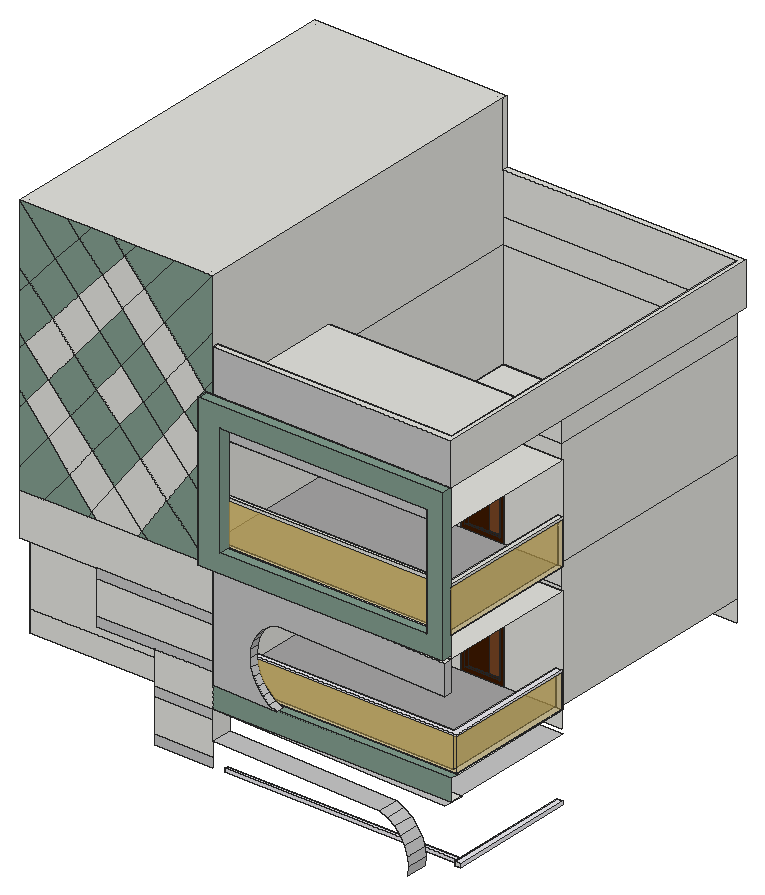
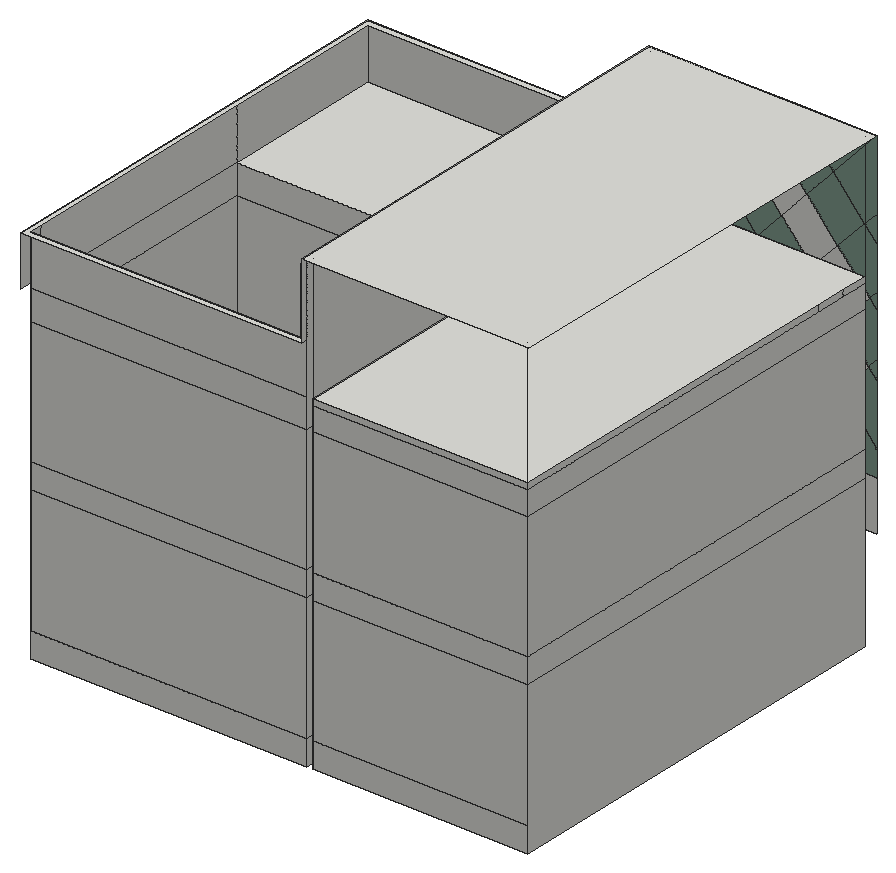
# SketchUp Ruby script. Lengths in inches.
U = 1.inch
M = Sketchup.active_model
def pt(a) = Geom::Point3d.new(a.map { |v| v * U })
def face(e, loops, mat)
  f = e.add_face(loops[0].map { |a| pt(a) })
  loops[1..].each { |l| e.add_face(l.map { |a| pt(a) }).erase! }
  f.material = f.back_material = mat if mat
  f
end
# faces: each face lists its corners as indices into pts; further lists are holes
def faces(e, pts, list, mat = nil) = list.each { |f| face(e, (f[0].is_a?(Array) ? f : [f]).map { |l| l.map { |i| pts[i] } }, mat) }
# xy, xz, yz: faces in a plane at the given z, y or x. An outline is a flat list of corners, or four numbers for a rectangle; further outlines are holes
def ring(l) = l.size == 4 ? [[l[0], l[1]], [l[2], l[1]], [l[2], l[3]], [l[0], l[3]]] : l.each_slice(2).to_a
def flat(e, list, mat, &to3) = list.each { |f| face(e, (f[0].is_a?(Array) ? f : [f]).map { |l| ring(l).map { |u, v| to3.(u, v) } }, mat) }
def xy(e, z, list, mat = nil) = flat(e, list, mat) { |x, y| [x, y, z] }
def xz(e, y, list, mat = nil) = flat(e, list, mat) { |x, z| [x, y, z] }
def yz(e, x, list, mat = nil) = flat(e, list, mat) { |y, z| [x, y, z] }
def lines(e, pts, list) = list.each { |a, b| e.add_line(pt(pts[a]), pt(pts[b])) }
# prism: a flat outline (further loops are holes) pulled along v
def prism(e, loops, v, mat = nil)
  f = face(e, loops, mat); d = Geom::Vector3d.new(v.map { |x| x * U })
  f.pushpull(f.normal.samedirection?(d) ? d.length : -d.length)
end
def box(e, o, s, mat = nil) = prism(e, [[o, [o[0] + s[0], o[1], o[2]], [o[0] + s[0], o[1] + s[1], o[2]], [o[0], o[1] + s[1], o[2]]]], [0, 0, s[2]], mat)
def at(x, y, z, deg = 0) = Geom::Transformation.translation(pt([x, y, z])) * Geom::Transformation.rotation(ORIGIN, Z_AXIS, deg.degrees)
def axes(o, x, y, z) = Geom::Transformation.new([*x, 0, *y, 0, *z, 0, *pt(o).to_a, 1])
def part(name) = M.definitions.add(name)
# library, detail: a bought-in or finely detailed component or shape, given as its bounding box
def library(name, o, s) = part(name).tap { |d| box(d.entities, o, s) }
def detail(e, o, s) = box(e.add_group.entities, o, s)
def put(e, d, t, mat = nil) = e.add_instance(d, t).tap { |i| i.material = mat if mat }
def group(e, t, mat = nil) = e.add_group.tap { |g| g.transformation = t; g.material = mat if mat }.entities
root = M.entities
M.materials.add("[Color B08]").color = [62, 25, 0]
M.materials.add("[Color H08]").color = [130, 158, 143]
M.materials.add("[Color M02]").color = [198, 198, 198]
M.materials.add("[Metal Silver]").color = [234, 233, 238]
M.materials.add("[Stone Vein Gray]").color = [166, 165, 165]
M.materials.add("[Translucent Glass Blue]").color = [201, 149, 0]
M.materials["[Translucent Glass Blue]"].alpha = 0.5
M.materials.add("[Translucent Glass Blue]1").color = [221, 188, 93]
M.materials["[Translucent Glass Blue]1"].alpha = 0.5
M.materials.add("[Wood Veneer 01]").color = [120, 70, 37]
c1 = part("Group\#2")
xy(c1.entities,0,[[0,0,48,4.9375]])
xy(c1.entities,3.28,[[23.77,0,25.1875,4.9375]])
xy(c1.entities,3.28,[[3.28,0,23.77,4.9375],[25.1875,0,44.72,4.9375]],"[Color B08]")
xy(c1.entities,56.72,[[23.77,0,25.1875,4.9375]])
xy(c1.entities,56.72,[[3.28,0,23.77,4.9375],[25.1875,0,44.72,4.9375]],"[Color B08]")
xy(c1.entities,60,[[0,0,48,4.9375]],"[Color B08]")
xz(c1.entities,0,[[[0,0,48,60],[3.28,3.28,44.72,56.72]],[23.77,3.28,25.1875,56.72]],"[Color B08]")
xz(c1.entities,4.9375,[[[0,0,48,60],[3.28,3.28,44.72,56.72]],[23.77,3.28,25.1875,56.72]],"[Color B08]")
xz(c1.entities,4.9375,[[3.28,3.28,23.77,56.72],[25.1875,3.28,44.72,56.72]],"[Translucent Glass Blue]")
yz(c1.entities,0,[[0,0,4.9375,60]],"[Color B08]")
yz(c1.entities,3.28,[[0,3.28,4.9375,56.72]],"[Color B08]")
yz(c1.entities,23.77,[[0,3.28,4.9375,56.72]],"[Color B08]")
yz(c1.entities,25.1875,[[0,3.28,4.9375,56.72]],"[Color B08]")
yz(c1.entities,44.72,[[0,3.28,4.9375,56.72]],"[Color B08]")
yz(c1.entities,48,[[0,0,4.9375,60]],"[Color B08]")
c2 = part("Group\#1")
xy(c2.entities,0,[[0,0,48,3.5]])
xy(c2.entities,4.73,[[4.73,0,28,3.5],[28,0,43.27,3.5]],"[Color B08]")
xy(c2.entities,79.27,[[4.73,0,28,3.5],[28,0,43.27,3.5]])
xy(c2.entities,84,[[0,0,48,3.5]],"[Color B08]")
xz(c2.entities,0,[[[0,0,48,84],[4.73,4.73,43.27,79.27]]],"[Color B08]")
xz(c2.entities,1.8125,[[8.85,40.5625,9.49,40.61,10.09,40.82,10.62,41.17,11.03,41.66,11.31,42.23,11.43,42.85,11.38,43.49,11.17,44.09,10.82,44.62,10.33,45.03,9.76,45.31,9.14,45.43,8.5,45.38,7.9,45.17,7.375,44.81,6.96,44.33,6.68,43.76,6.5625,43.14,6.61,42.5,6.82,41.9,7.17,41.375,7.66,40.96,8.23,40.68]],"[Metal Silver]")
xz(c2.entities,3.5,[[[0,0,48,84],[4.73,4.73,43.27,79.27]],[[4.73,4.73,28,79.27],[8.85,40.5625,8.23,40.68,7.66,40.96,7.17,41.375,6.82,41.9,6.61,42.5,6.5625,43.14,6.68,43.76,6.96,44.33,7.375,44.81,7.9,45.17,8.5,45.38,9.14,45.43,9.76,45.31,10.33,45.03,10.82,44.62,11.17,44.09,11.38,43.49,11.43,42.85,11.31,42.23,11.03,41.66,10.62,41.17,10.09,40.82,9.49,40.61]]],"[Color B08]")
xz(c2.entities,3.5,[[8.85,40.5625,8.23,40.68,7.66,40.96,7.17,41.375,6.82,41.9,6.61,42.5,6.5625,43.14,6.68,43.76,6.96,44.33,7.375,44.81,7.9,45.17,8.5,45.38,9.14,45.43,9.76,45.31,10.33,45.03,10.82,44.62,11.17,44.09,11.38,43.49,11.43,42.85,11.31,42.23,11.03,41.66,10.62,41.17,10.09,40.82,9.49,40.61]],"[Metal Silver]")
xz(c2.entities,3.5,[[28,4.73,43.27,79.27]],"[Wood Veneer 01]")
yz(c2.entities,0,[[0,0,3.5,84]],"[Color B08]")
yz(c2.entities,4.73,[[0,4.73,3.5,79.27]],"[Color B08]")
yz(c2.entities,43.27,[[0,4.73,3.5,79.27]],"[Color B08]")
yz(c2.entities,48,[[0,0,3.5,84]],"[Color B08]")
p = [[8.23,3.5,40.68],[8.85,3.5,40.5625],[8.85,1.8125,40.5625],[8.23,1.8125,40.68],[9.49,3.5,40.61],[9.49,1.8125,40.61],
  [10.09,3.5,40.82],[10.09,1.8125,40.82],[7.66,3.5,40.96],[7.66,1.8125,40.96],[10.62,3.5,41.17],[10.62,1.8125,41.17],
  [7.17,3.5,41.375],[7.17,1.8125,41.375],[11.03,3.5,41.66],[11.03,1.8125,41.66],[6.82,3.5,41.9],[6.82,1.8125,41.9],
  [11.31,3.5,42.23],[11.31,1.8125,42.23],[6.61,3.5,42.5],[6.61,1.8125,42.5],[11.43,3.5,42.85],[11.43,1.8125,42.85],
  [6.5625,3.5,43.14],[6.5625,1.8125,43.14],[11.38,3.5,43.49],[11.38,1.8125,43.49],[6.68,3.5,43.76],[6.68,1.8125,43.76],
  [11.17,3.5,44.09],[11.17,1.8125,44.09],[6.96,3.5,44.33],[6.96,1.8125,44.33],[10.82,3.5,44.62],[10.82,1.8125,44.62],
  [7.375,3.5,44.81],[7.375,1.8125,44.81],[10.33,3.5,45.03],[10.33,1.8125,45.03],[7.9,3.5,45.17],[7.9,1.8125,45.17],
  [9.76,3.5,45.31],[9.76,1.8125,45.31],[8.5,3.5,45.38],[8.5,1.8125,45.38],[9.14,3.5,45.43],[9.14,1.8125,45.43]]
faces(c2.entities,p,[[0,1,2,3],[1,4,5,2],[4,6,7,5],[8,0,3,9],[6,10,11,7],[12,8,9,13],[10,14,15,11],[16,12,13,17],
  [14,18,19,15],[20,16,17,21],[18,22,23,19],[24,20,21,25],[22,26,27,23],[28,24,25,29],[26,30,31,27],[32,28,29,33],
  [30,34,35,31],[36,32,33,37],[34,38,39,35],[40,36,37,41],[38,42,43,39],[44,40,41,45],[42,46,47,43],[46,44,45,47]],"[Metal Silver]")
xy(root,322.25,[[347.4375,299.125,395.4375,305.125]])
xy(root,345,[[554.1875,155.45,547.7,155.68,547.7,299.125,554.1875,299.125],[285.75,159.75,547.7,163.37]])
xy(root,349.125,[[554.1875,155.45,554.1875,299.125,547.7,299.125,547.7,155.68],[285.75,159.75,547.7,163.37]],"[Metal Silver]")
xy(root,381,[[439.75,299.125,487.75,305.125]])
xy(root,382.25,[[347.4375,299.125,395.4375,305.125]])
xy(root,384.9,[[478.91,135.35,285.75,142.1875,286.55,164.92,479.71,158.09]],"[Color M02]")
xy(root,417,[[285.75,142.1875,286.55,164.92,554.1875,155.45,554.1875,142.1875]])
xy(root,417,[[554.1875,132.6875,554.99,155.42,554.1875,155.45,554.1875,142.1875,285.75,142.1875],[285.75,142.1875,285.75,299.125,554.1875,299.125,554.1875,155.45,286.55,164.92]],"[Color M02]")
xy(root,441,[[359.42,139.58,285.75,142.1875,359.51,142.1875],[285.75,142.1875,285.75,155.78,546.37,155.78,546.37,299.125,552.75,299.125,552.75,151.18,286.07,151.18],[285.75,142.1875,359.51,142.1875,359.74,148.57,286.07,151.18],[552.75,151.18,554.1875,299.125],[285.75,305.125,548.75,550.1875]])
xy(root,441,[[359.51,142.1875,554.1875,142.1875,554.1875,151.18,286.07,151.18,359.74,148.57]],"[Color H08]")
xy(root,441,[[285.75,155.78,546.37,155.78,546.37,299.125,487.75,299.125,487.75,305.125,439.75,305.125,439.75,299.125,285.75,299.125]],"[Stone Vein Gray]")
xy(root,469.3,[[358.47,299.125,406.47,305.125]])
xy(root,478.1875,[[285.75,142.1875,285.75,155.78,546.37,155.78,546.37,299.125,552.75,299.125,552.75,151.18,286.07,151.18]])
xy(root,480.8125,[[285.75,142.1875,286.07,151.18,552.75,151.18,552.75,299.125,546.37,299.125,546.37,155.78,285.75,155.78]],"[Metal Silver]")
xy(root,525,[[439.75,299.125,487.75,305.125]])
xy(root,527.64,[[554.1875,132.6875,359.42,139.58,359.74,148.57,554.51,141.68]],"[Color M02]")
xy(root,529.3,[[358.47,299.125,406.47,305.125]])
xy(root,561,[[554.1875,132.6875,554.51,141.68,540.22,142.1875,285.75,142.1875],[285.75,142.1875,285.75,299.125,554.1875,299.125,554.1875,142.1875,540.22,142.1875,286.07,151.18],[285.75,142.1875,540.22,142.1875,286.07,151.18]])
xy(root,564.5,[[278.75,130.5,554.1875,142.1875]],"[Color H08]")
xy(root,585,[[285.75,142.1875,285.75,146.18,548.53,146.18,548.53,299.125,554.1875,299.125,554.1875,142.1875],[75,148.1875,279.75,550.1875],[285.75,305.125,548.75,550.1875]])
xy(root,585,[[303.46,130.5,535.58,142.1875]],"[Color H08]")
xy(root,585,[[285.75,146.18,548.53,146.18,548.53,299.125,487.75,299.125,487.75,305.125,439.75,305.125,439.75,299.125,285.75,299.125]],"[Stone Vein Gray]")
xy(root,610.67,[[357.4375,299.125,405.4375,305.125]])
xy(root,633,[[285.75,142.1875,285.75,146.18,548.53,146.18,548.53,299.125,554.1875,299.125,554.1875,142.1875]])
xy(root,636.0625,[[285.75,142.1875,554.1875,142.1875,554.1875,299.125,548.53,299.125,548.53,146.18,285.75,146.18]])
xy(root,669,[[439.75,299.125,487.75,305.125]])
xy(root,670.67,[[357.4375,299.125,405.4375,305.125]])
xy(root,693.3125,[[285.75,142.1875,554.1875,299.125]])
xy(root,711.16,[[303.46,130.5,535.58,142.1875]],"[Color H08]")
xy(root,727.5,[[75,148.1875,279.75,550.1875]])
xy(root,733.5,[[75,148.1875,279.75,550.1875],[285.75,149.25,548.75,305.125]])
xy(root,733.5,[[278.75,130.5,554.1875,142.1875]],"[Color H08]")
xy(root,781.5,[[285.75,142.1875,554.1875,142.1875,554.1875,556.1875,285.75,556.1875,285.75,550.1875,548.75,550.1875,548.75,149.25,285.75,149.25]])
xy(root,853.5,[[69,142.1875,285.75,556.1875]])
xz(root,130.5,[[[278.75,564.5,554.1875,733.5],[303.46,585,535.58,711.16]]],"[Color H08]")
xz(root,142.1875,[[220.2,368.75,285.75,405.77],[220.2,416.8125,285.75,453.83],[155.14,464.875,285.75,501.89],[69,512.9375,285.75,561],[155.14,561,201.21,561,206.51,568.59,176.11,601.9,149.83,567.23],
  [285.75,561,554.1875,564.5],[278.75,564.5,554.1875,585],[149.83,567.23,176.11,601.9,151.23,629.16,124.87,596.5],[206.51,568.59,234.39,608.49,204.97,639.98,176.11,601.9],[278.75,585,285.75,585,285.75,693.3125,303.46,693.3125,303.46,711.16,554.1875,711.16,554.1875,733.5,278.75,733.5],
  [285.75,585,303.46,633],[535.58,585,554.1875,633],[124.87,596.5,151.23,629.16,126.51,656.24,100.9375,624.5625],[234.39,608.49,258.56,643.08,230.73,673.97,204.97,639.98],[100.9375,624.5625,126.51,656.24,101.33,683.83,76.17,653.61],
  [285.75,633,303.46,636.0625],[303.46,633,535.58,636.0625],[535.58,633,554.1875,636.0625],[258.56,643.08,278.75,671.98,278.75,678.83,254.79,705.71,230.73,673.97],[180.83,665.83,207.88,699.34,183.3125,726.61,155.84,692.58],
  [101.33,683.83,130.87,719.31,105.46,746.51,75.38,712.26],[535.58,693.3125,554.1875,711.16],[254.79,705.71,277.2,735.28,256.3,759.32,232.87,730.29],[130.87,719.31,159.22,753.35,135.05,780.18,105.46,746.51],[232.87,730.29,256.3,759.32,232.15,787.1,208.43,757.71],
  [159.22,753.35,184.86,784.15,161.53,810.32,135.05,780.18],[208.43,757.71,232.15,787.1,209.25,813.45,184.86,784.15],[184.86,784.15,209.25,813.45,186.88,839.18,161.53,810.32]])
xz(root,142.1875,[[285.75,417,554.1875,441],[69,561,96.21,561,124.87,596.5,100.9375,624.5625,69,585],[96.21,561,145.11,561,149.83,567.23,124.87,596.5],[145.11,561,155.14,561,149.83,567.23],[201.21,561,213.44,561,206.51,568.59],
  [213.44,561,278.75,561,234.39,608.49,206.51,568.59],[278.75,561,285.75,561,285.75,564.5,278.75,564.5,278.75,620.67,258.56,643.08,234.39,608.49],[69,585,100.9375,624.5625,76.17,653.61,69,645],[176.11,601.9,204.97,639.98,180.83,665.83,151.23,629.16],[278.75,620.67,278.75,671.98,258.56,643.08],
  [151.23,629.16,180.83,665.83,155.84,692.58,126.51,656.24],[285.75,636.0625,303.46,693.3125],[535.58,636.0625,554.1875,693.3125],[204.97,639.98,230.73,673.97,207.88,699.34,180.83,665.83],[69,645,76.17,653.61,69,662.02],
  [76.17,653.61,101.33,683.83,75.38,712.26,69,705,69,662.02],[126.51,656.24,155.84,692.58,130.87,719.31,101.33,683.83],[230.73,673.97,254.79,705.71,232.87,730.29,207.88,699.34],[278.75,678.83,278.75,733.5,277.2,735.28,254.79,705.71],[155.84,692.58,183.3125,726.61,159.22,753.35,130.87,719.31],
  [207.88,699.34,232.87,730.29,208.43,757.71,183.3125,726.61],[69,705,75.38,712.26,69,719.25],[75.38,712.26,105.46,746.51,79.67,774.12,69,761.97,69,719.25],[183.3125,726.61,208.43,757.71,184.86,784.15,159.22,753.35],[278.75,733.5,285.75,733.5,285.75,746.56,277.2,735.28],
  [277.2,735.28,285.75,746.56,285.75,795.8,256.3,759.32],[105.46,746.51,135.05,780.18,109.71,808.31,79.67,774.12],[256.3,759.32,285.75,795.8,285.75,853.5,232.15,787.1],[69,761.97,79.67,774.12,69,785.54],[79.67,774.12,109.71,808.31,69,853.5,69,785.54],
  [135.05,780.18,161.53,810.32,136.32,838.6,109.71,808.31],[232.15,787.1,285.75,853.5,242.6,853.5,209.25,813.45],[109.71,808.31,136.32,838.6,123.04,853.5,69,853.5],[161.53,810.32,186.88,839.18,174.43,853.5,149.41,853.5,136.32,838.6],[209.25,813.45,242.6,853.5,199.46,853.5,186.88,839.18],
  [136.32,838.6,149.41,853.5,123.04,853.5],[186.88,839.18,199.46,853.5,174.43,853.5]],"[Color H08]")
xz(root,142.1875,[[220.2,357.7,285.75,368.75],[220.2,405.77,285.75,416.8125],[155.14,453.83,285.75,464.875],[155.14,501.89,285.75,512.9375],[303.46,693.3125,535.58,711.16],
  [285.75,733.5,554.1875,781.5]],"[Color M02]")
xz(root,142.1875,[[303.46,585,535.58,633]],"[Translucent Glass Blue]1")
xz(root,146.18,[[285.75,633,548.53,636.0625]])
xz(root,146.18,[[285.75,585,548.53,633]],"[Translucent Glass Blue]1")
xz(root,148.1875,[[75,417,279.75,441],[75,441,279.75,561],[75,561,279.75,585],[75,585,279.75,705],[75,705,279.75,727.5],
  [75,727.5,279.75,733.5]])
xz(root,149.25,[[285.75,733.5,548.75,781.5]])
xz(root,151.18,[[286.07,478.1875,552.75,480.8125]],"[Metal Silver]")
xz(root,151.18,[[286.07,441,552.75,478.1875]],"[Translucent Glass Blue]1")
xz(root,155.78,[[285.75,478.1875,546.37,480.8125]],"[Metal Silver]")
xz(root,155.78,[[285.75,441,546.37,478.1875]],"[Translucent Glass Blue]1")
xz(root,159.75,[[285.75,345,547.7,349.125]],"[Metal Silver]")
xz(root,163.37,[[285.75,345,547.7,349.125]],"[Metal Silver]")
xz(root,299.125,[[547.7,345,554.1875,349.125],[[285.75,441,439.75,441,439.75,525,487.75,525,487.75,441,546.37,441,546.37,480.8125,552.75,480.8125,552.75,478.1875,554.1875,478.1875,554.1875,561,285.75,561],[358.47,469.3,406.47,529.3]],[546.37,441,552.75,478.1875],[552.75,441,554.1875,478.1875],[546.37,478.1875,552.75,480.8125],
  [[285.75,585,439.75,585,439.75,669,487.75,669,487.75,585,548.53,585,548.53,636.0625,554.1875,636.0625,554.1875,693.3125,285.75,693.3125],[357.4375,610.67,405.4375,670.67]],[548.53,585,554.1875,633],[548.53,633,554.1875,636.0625]])
xz(root,305.125,[[285.75,417,548.75,441],[[285.75,441,285.75,561,548.75,561,548.75,441,487.75,441,487.75,525,439.75,525,439.75,441],[358.47,469.3,406.47,529.3]],[285.75,561,548.75,585],[[285.75,585,285.75,705,548.75,705,548.75,585,487.75,585,487.75,669,439.75,669,439.75,585],[357.4375,610.67,405.4375,670.67]],[285.75,705,548.75,733.5]])
xz(root,550.1875,[[75,417,279.75,441],[285.75,417,548.75,441],[75,441,279.75,561],[285.75,441,548.75,561],[75,561,279.75,585],
  [285.75,561,548.75,585],[75,585,279.75,705],[285.75,585,548.75,705],[75,705,279.75,727.5],[285.75,705,548.75,733.5],
  [75,727.5,279.75,733.5],[285.75,733.5,548.75,781.5]])
yz(root,75,[[148.1875,417,550.1875,561],[148.1875,561,550.1875,585],[148.1875,585,550.1875,705],[148.1875,705,550.1875,727.5],[148.1875,727.5,175.05,733.5],
  [175.05,727.5,203.8,733.5],[203.8,727.5,550.1875,733.5]])
yz(root,278.75,[[130.5,564.5,142.1875,585],[130.5,585,142.1875,733.5]],"[Color H08]")
yz(root,279.75,[[148.1875,417,550.1875,441],[148.1875,441,550.1875,561],[148.1875,561,550.1875,585],[148.1875,585,550.1875,705],[148.1875,705,550.1875,727.5],
  [148.1875,727.5,550.1875,733.5]])
yz(root,285.75,[[159.75,345,163.37,349.125],[305.125,417,550.1875,441],[142.1875,441,155.78,478.1875],[155.78,441,299.125,441,299.125,561,142.1875,561,142.1875,480.8125,155.78,480.8125],[305.125,441,550.1875,561],
  [142.1875,478.1875,155.78,480.8125],[305.125,561,550.1875,585],[142.1875,585,146.18,633],[146.18,585,299.125,585,299.125,693.3125,142.1875,693.3125,142.1875,636.0625,146.18,636.0625],[305.125,585,550.1875,705],
  [142.1875,633,146.18,636.0625],[305.125,705,550.1875,705,550.1875,853.5,142.1875,853.5,142.1875,781.5,149.25,781.5,149.25,733.5,305.125,733.5],[142.1875,733.5,149.25,781.5],[550.1875,781.5,556.1875,853.5]])
yz(root,303.46,[[130.5,585,142.1875,711.16]],"[Color H08]")
yz(root,347.4375,[[299.125,322.25,305.125,382.25]])
yz(root,357.4375,[[299.125,610.67,305.125,670.67]])
yz(root,358.47,[[299.125,469.3,305.125,529.3]])
yz(root,395.4375,[[299.125,322.25,305.125,382.25]])
yz(root,405.4375,[[299.125,610.67,305.125,670.67]])
yz(root,406.47,[[299.125,469.3,305.125,529.3]])
yz(root,439.75,[[299.125,441,305.125,525],[299.125,585,305.125,669]])
yz(root,487.75,[[299.125,441,305.125,525],[299.125,585,305.125,669]])
yz(root,535.58,[[130.5,585,142.1875,711.16]],"[Color H08]")
yz(root,546.37,[[155.78,478.1875,299.125,480.8125]],"[Metal Silver]")
yz(root,546.37,[[155.78,441,299.125,478.1875]],"[Translucent Glass Blue]1")
yz(root,547.7,[[155.68,345,159.75,349.125],[159.75,345,163.37,349.125]])
yz(root,547.7,[[163.37,345,299.125,349.125]],"[Metal Silver]")
yz(root,548.53,[[146.18,633,299.125,636.0625]])
yz(root,548.53,[[146.18,585,299.125,633]],"[Translucent Glass Blue]1")
yz(root,548.75,[[305.125,441,550.1875,585],[305.125,585,550.1875,705],[305.125,705,550.1875,733.5],[149.25,733.5,305.125,781.5],[305.125,733.5,538.375,781.5],
  [538.375,733.5,550.1875,781.5]])
yz(root,552.75,[[151.18,478.1875,299.125,480.8125]],"[Metal Silver]")
yz(root,552.75,[[151.18,441,299.125,478.1875]],"[Translucent Glass Blue]1")
yz(root,554.1875,[[142.1875,633,299.125,636.0625],[142.1875,733.5,556.1875,781.5]])
yz(root,554.1875,[[130.5,564.5,142.1875,733.5]],"[Color H08]")
yz(root,554.1875,[[155.45,345,299.125,349.125]],"[Metal Silver]")
yz(root,554.1875,[[142.1875,585,299.125,633]],"[Translucent Glass Blue]1")
p = [[512.51,134.16,340.95],[513.32,156.9,340.95],[512.24,156.9375,331.12],[511.4375,134.2,331.12],[511.4375,134.2,350.78],[512.24,156.9375,350.78],
  [554.1875,155.45,345],[547.7,155.68,345],[547.7,155.68,349.125],[554.1875,155.45,349.125],[508.27,134.3125,360.15],[509.07,157.05,360.15],
  [503.15,134.49,368.62],[503.95,157.23,368.62],[496.32,134.74,375.78],[497.125,157.47,375.78],[488.11,135.03,381.29],[488.92,157.76,381.29],
  [478.91,135.35,384.9],[479.71,158.09,384.9],[285.75,142.1875,417],[286.55,164.92,417],[286.55,164.92,384.9],[285.75,142.1875,384.9],
  [285.75,142.1875,405.77],[285.75,142.1875,416.8125],[351.0625,139.875,523.5],[359.42,139.58,527.64],[554.1875,132.6875,527.64],[554.1875,132.6875,561],
  [285.75,142.1875,561],[285.75,142.1875,512.9375],[285.75,142.1875,501.89],[285.75,142.1875,480.8125],[285.75,142.1875,478.1875],[285.75,142.1875,464.875],
  [285.75,142.1875,453.83],[285.75,142.1875,441],[359.42,139.58,441],[351.0625,139.875,445.14],[343.71,140.14,450.875],[337.65,140.35,457.97],
  [333.14,140.51,466.13],[330.36,140.61,475.04],[329.42,140.64,484.32],[330.36,140.61,493.6],[333.14,140.51,502.51],[337.65,140.35,510.67],
  [343.71,140.14,517.76],[359.74,148.57,441],[351.38,148.87,445.14],[359.51,142.1875,441],[359.74,148.57,527.64],[351.38,148.87,523.5],
  [344.03,149.13,517.76],[337.97,149.35,510.67],[333.46,149.5,502.51],[330.68,149.6,493.6],[329.74,149.64,484.32],[330.68,149.6,475.04],
  [333.46,149.5,466.13],[337.97,149.35,457.97],[344.03,149.13,450.875],[286.07,151.18,441],[286.07,151.18,478.1875],[286.07,151.18,480.8125],
  [286.07,151.18,561],[540.22,142.1875,561],[554.51,141.68,561],[554.51,141.68,527.64],[285.75,142.1875,705],[285.75,299.125,705],
  [285.75,299.125,693.3125],[75,148.1875,733.5],[75,148.1875,853.5],[279.75,148.1875,733.5],[279.75,148.1875,853.5],[75,550.1875,733.5],
  [75,550.1875,853.5],[279.75,550.1875,733.5],[279.75,550.1875,853.5],[285.75,155.78,441],[279.75,155.78,441]]
faces(root,p,[[0,1,2,3],[4,5,1,0],[10,11,5,4],[12,13,11,10],[14,15,13,12],[16,17,15,14],[18,19,17,16],[26,27,28,29,30,31,32,33,34,35,36,37,38,39,40,41,42,43,44,45,46,47,48],
  [49,50,39,38,51],[52,53,54,55,56,57,58,59,60,61,62,50,49,63,64,65,66,67,68,69],[50,62,40,39],[62,61,41,40],[61,60,42,41],[60,59,43,42],[59,58,44,43],[58,57,45,44],
  [57,56,46,45],[56,55,47,46],[55,54,48,47],[54,53,26,48],[53,52,27,26],[69,68,29,28]],"[Color M02]")
faces(root,p,[[6,7,8,9],[20,21,22,23,24,25],[63,37,36,35,34,64],[64,34,33,65],[66,65,33,32,31,30]])
lines(root,p,[[70,71],[72,71],[73,74],[75,76],[77,78],[79,80],[81,82]])
put(root,c1,at(347.4375,299.125,322.25))
put(root,c2,at(439.75,299.125,441))
put(root,c1,at(358.47,299.125,469.3))
put(root,c2,at(439.75,299.125,585))
put(root,c1,at(357.4375,299.125,610.67))
